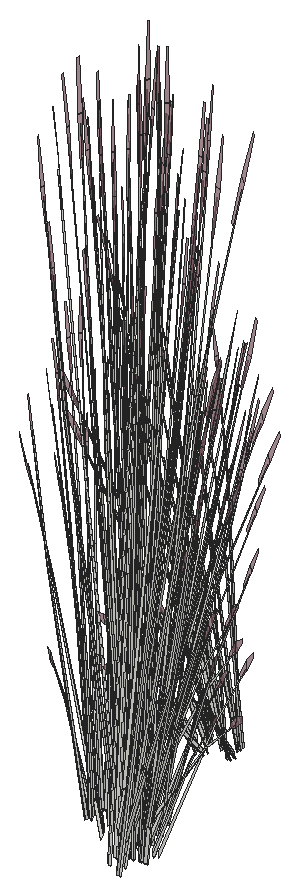
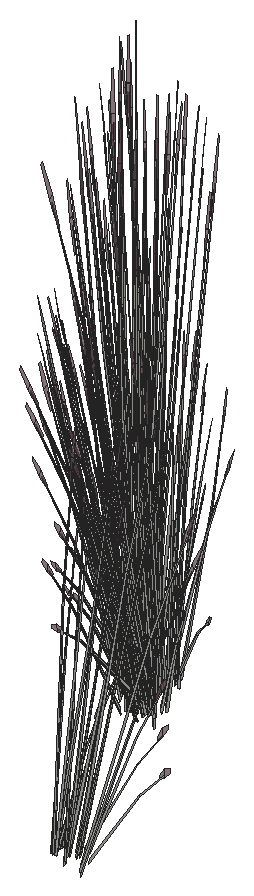
# SketchUp Ruby script. Lengths in inches.
U = 1.inch
M = Sketchup.active_model
def pt(a) = Geom::Point3d.new(a.map { |v| v * U })
def face(e, loops, mat)
  f = e.add_face(loops[0].map { |a| pt(a) })
  loops[1..].each { |l| e.add_face(l.map { |a| pt(a) }).erase! }
  f.material = f.back_material = mat if mat
  f
end
# faces: each face lists its corners as indices into pts; further lists are holes
def faces(e, pts, list, mat = nil) = list.each { |f| face(e, (f[0].is_a?(Array) ? f : [f]).map { |l| l.map { |i| pts[i] } }, mat) }
# xy, xz, yz: faces in a plane at the given z, y or x. An outline is a flat list of corners, or four numbers for a rectangle; further outlines are holes
def ring(l) = l.size == 4 ? [[l[0], l[1]], [l[2], l[1]], [l[2], l[3]], [l[0], l[3]]] : l.each_slice(2).to_a
def flat(e, list, mat, &to3) = list.each { |f| face(e, (f[0].is_a?(Array) ? f : [f]).map { |l| ring(l).map { |u, v| to3.(u, v) } }, mat) }
def xy(e, z, list, mat = nil) = flat(e, list, mat) { |x, y| [x, y, z] }
def xz(e, y, list, mat = nil) = flat(e, list, mat) { |x, z| [x, y, z] }
def yz(e, x, list, mat = nil) = flat(e, list, mat) { |y, z| [x, y, z] }
def lines(e, pts, list) = list.each { |a, b| e.add_line(pt(pts[a]), pt(pts[b])) }
# prism: a flat outline (further loops are holes) pulled along v
def prism(e, loops, v, mat = nil)
  f = face(e, loops, mat); d = Geom::Vector3d.new(v.map { |x| x * U })
  f.pushpull(f.normal.samedirection?(d) ? d.length : -d.length)
end
def box(e, o, s, mat = nil) = prism(e, [[o, [o[0] + s[0], o[1], o[2]], [o[0] + s[0], o[1] + s[1], o[2]], [o[0], o[1] + s[1], o[2]]]], [0, 0, s[2]], mat)
def at(x, y, z, deg = 0) = Geom::Transformation.translation(pt([x, y, z])) * Geom::Transformation.rotation(ORIGIN, Z_AXIS, deg.degrees)
def axes(o, x, y, z) = Geom::Transformation.new([*x, 0, *y, 0, *z, 0, *pt(o).to_a, 1])
def part(name) = M.definitions.add(name)
# library, detail: a bought-in or finely detailed component or shape, given as its bounding box
def library(name, o, s) = part(name).tap { |d| box(d.entities, o, s) }
def detail(e, o, s) = box(e.add_group.entities, o, s)
def put(e, d, t, mat = nil) = e.add_instance(d, t).tap { |i| i.material = mat if mat }
def group(e, t, mat = nil) = e.add_group.tap { |g| g.transformation = t; g.material = mat if mat }.entities
root = M.entities
M.materials.add("LightPink_Translucent").color = [144, 107, 117]
M.materials["LightPink_Translucent"].alpha = 0.75
c1 = part("blade")
p = [[2.15,0.21,22],[0,0.17,0],[0.09,0.45,0],[2.18,0.31,22],[2.29,0.31,22],[0.38,0.45,0],
  [2.48,0.24,33],[2.49,0.24,33],[2.48,0.22,33]]
faces(c1.entities,p,[[0,1,2,3],[4,5,2,3],[6,3,4,7],[8,0,3,6]])
c2 = part("seeds")
p = [[0.3,-0.1,1.38],[-0.01,-0.03,1.59],[-0.01,-0.03,0.03],[0.14,-0.07,-0.07],[0.29,-0.03,3],[0.15,0.01,3.11]]
faces(c2.entities,p,[[0,1,2,3],[1,0,4,5]],"LightPink_Translucent")
c3 = part("blade with seeds")
put(c3.entities,c1,at(0,0,0))
put(c3.entities,c2,axes([2.4,0.25,30.99],[1.5799,-0.05474,1.17369],[-0.12525,1.92788,0.29478],[-0.07173,-0.02425,1.56792]))
put(root,c3,axes([406.07,308.69,4.74],[-0.08839,-0.48081,-0.26641],[0.35106,-0.13653,0.26641],[-0.07077,-0.05545,1.19518]))
put(root,c3,axes([406.53,308.66,5.13],[0.40434,-0.14646,0.15172],[0.09984,0.54504,0.30174],[-0.03606,-0.07941,1.3795]))
put(root,c3,axes([407.36,306.6,5.29],[0.37992,-0.36634,-0.25022],[0.25264,0.51764,-0.43002],[0.09374,0.05257,1.37348]))
put(root,c3,axes([408.87,307.57,6.89],[0.31272,0.15393,-0.30456],[-0.09121,0.44909,0.39319],[0.1259,-0.04118,0.75234]))
put(root,c3,axes([405.98,308.9,4.74],[-0.35217,-0.2759,-0.427],[0.2105,-0.49473,0],[-0.08021,-0.06284,1.35453]))
put(root,c3,axes([408.32,305.63,4.74],[0.35217,0.2759,-0.427],[-0.2105,0.49473,0],[0.08021,0.06284,1.35453]))
put(root,c3,axes([405.19,306.86,6.89],[-0.31272,-0.15393,-0.30456],[0.09121,-0.44909,0.39319],[-0.1259,0.04118,0.75234]))
put(root,c3,axes([407.65,307.2,4.9],[0.42099,0,0],[0,0.57126,0],[0,0,1.5343]))
put(root,c3,axes([406.93,307.92,5.29],[-0.37992,0.36634,-0.25022],[-0.25264,-0.51764,-0.43002],[-0.09374,-0.05257,1.37348]))
put(root,c3,axes([407.77,305.87,5.13],[-0.40434,0.14646,0.15172],[-0.09984,-0.54504,0.30174],[0.03606,0.07941,1.3795]))
put(root,c3,axes([408.02,307.01,6.33],[-0.15608,0.0125,1.47384],[0.10354,-0.54165,0.11917],[0.22242,0.0335,0.63005]))
put(root,c3,axes([408.22,305.84,4.74],[0.08839,0.48081,-0.26641],[-0.35106,0.13653,0.26641],[0.07077,0.05545,1.19518]))
put(root,c3,axes([408.82,307.76,7.07],[0.1382,0.37624,0.0553],[-0.25202,0.18416,0.43534],[0.11109,-0.03633,0.66383]))
put(root,c3,axes([407.51,306.91,5.05],[-0.4756,-0.11626,0.42311],[0.09679,-0.6566,0.16603],[0.0695,0.0634,1.46899]))
put(root,c3,axes([408.8,307.625,7.07],[-0.10631,0.50312,0.41282],[-0.34951,-0.17204,0.34039],[0.13745,-0.03024,0.85423]))
put(root,c3,axes([407.13,308.53,4.9],[-0.12277,-0.47573,0],[0.35059,-0.1666,0],[0,0,1.32759]))
put(root,c3,axes([406.9,308.08,5.25],[-0.07259,0.49245,0.12452],[-0.35466,-0.08548,-0.35559],[-0.06454,-0.05057,1.09]))
put(root,c3,axes([405.52,306.81,7.34],[0.31272,0.15393,0.30456],[-0.09121,0.44909,-0.39319],[-0.1259,0.04118,0.75234]))
put(root,c3,axes([407.59,308.47,4.88],[0.39505,-0.18722,-0.1651],[0.13882,0.53931,0.00007],[0.04361,-0.02069,1.49552]))
put(root,c3,axes([407.73,308.69,5.13],[0.1087,-0.54839,0.15172],[0.39778,0.15519,0.30174],[-0.06871,0.00267,1.3795]))
put(root,c3,axes([407.64,307.45,4.9],[0.26266,0.35642,0],[-0.26266,0.35642,0],[0,0,1.45569]))
put(root,c3,axes([406.15,306.78,5.875],[0.10696,-0.07982,1.52275],[0.03688,0.55733,0.11917],[-0.23167,0.07395,0.54424]))
put(root,c3,axes([408.35,307.29,5.13],[-0.29564,-0.40194,0.15172],[0.29793,-0.38985,0.30174],[-0.03265,0.08208,1.3795]))
put(root,c3,axes([407.8,306.6875,4.77],[0.39143,0.09047,-0.53624],[-0.0826,0.55804,-0.14074],[0.11681,0.06762,1.18365]))
put(root,c3,axes([409.53,307.66,5.38],[-0.23249,0.0911,0.9878],[0.10944,-0.37648,0.72577],[0.12334,0.02576,0.21757]))
put(root,c3,axes([407.05,308.75,4.89],[-0.37935,-0.24773,0],[0.18257,-0.51475,0],[0,0,1.39928]))
put(root,c3,axes([407.36,308.09,5.12],[-0.36743,-0.44413,-0.21665],[0.30918,-0.49872,0.47412],[-0.09894,0.05195,1.44665]))
put(root,c3,axes([406.39,308.94,5.13],[0.35217,0.2759,0.427],[-0.2105,0.49473,0],[-0.08021,-0.06284,1.35453]))
put(root,c3,axes([407.63,307.03,5.34],[0.18257,-0.49721,0.38476],[0.37935,0.23929,-0.18517],[0,0.11462,1.23533]))
put(root,c3,axes([409.42,309.25,7.05],[-0.03403,-0.04831,1.5255],[0.07443,-0.51782,-0.14414],[0.13402,-0.03308,0.26996]))
put(root,c3,axes([405,307.15,7.05],[-0.06145,0.07164,1.50452],[0.00523,0.52344,-0.23794],[-0.14085,0.06807,0.12066]))
put(root,c3,axes([407.56,307.32,4.97],[0,0.63816,-0.04848],[-0.47052,0,0],[0,0.02005,1.54256]))
put(root,c3,axes([405.41,307.08,7.03],[-0.10194,0.50193,-0.43945],[-0.34951,-0.17204,-0.34039],[-0.14072,0.04602,0.84085]))
put(root,c3,axes([405.39,306.65,7.33],[0.18933,0.49965,-0.10458],[-0.33602,0.24554,-0.58045],[-0.1416,0.06592,0.88199]))
put(root,c3,axes([407.6,306.86,4.9],[0.22605,0.46315,-0.38476],[-0.34239,0.32614,0.18517],[0.07315,0.05731,1.23533]))
put(root,c3,axes([409.13,308.82,6.38],[-0.07202,-0.46385,-0.03003],[0.3404,-0.10664,-0.13615],[0.07108,0.02941,0.44908]))
put(root,c3,axes([406.19,309.23,5.04],[-0.23526,0.55293,0],[-0.3936,-0.30836,-0.44382],[-0.08964,-0.07023,1.40792]))
put(root,c3,axes([408.25,308.81,7.33],[0.02015,-0.56117,-0.10458],[0.38148,0.01534,-0.58045],[0.14692,0.03898,0.88199]))
put(root,c3,axes([408.59,307.31,5.13],[0,-0.5518,0.427],[0.42099,0,0],[0,0.12568,1.35453]))
put(root,c3,axes([407.54,307.72,5.34],[0.40861,-0.03406,0.38476],[0.03695,0.56543,-0.18517],[-0.07315,0.05731,1.23533]))
put(root,c3,axes([407.79,307.15,5.25],[0.35059,-0.16092,0.12452],[0.12277,0.45952,-0.35559],[0,0.10113,1.09]))
put(root,c3,axes([408.1875,308.59,7.34],[-0.2141,-0.34548,0.30456],[0.24447,-0.32704,-0.39319],[0.12421,0.04976,0.75234]))
put(root,c3,axes([407.17,308,4.9],[-0.40861,0.03406,-0.38476],[-0.03695,-0.56543,0.18517],[-0.07315,0.05731,1.23533]))
put(root,c3,axes([409.1,308.27,5.23],[-0.09062,-0.13571,1.22981],[0.11791,-0.44895,-0.26449],[0.18335,0.06082,0.52581]))
put(root,c3,axes([407.48,308.76,4.9],[0.37935,0.24773,0],[-0.18257,0.51475,0],[0,0,1.5046]))
put(root,c3,axes([408.58,308.47,7.05],[0.08072,-0.00933,1.50452],[0.22141,-0.42869,-0.23794],[0.14358,0.05659,0.12066]))
put(root,c3,axes([407.63,309.31,4.89],[-0.23233,-0.55486,-0.04422],[0.3936,-0.30836,0.44382],[-0.09699,0.05283,1.40722]))
put(root,c3,axes([407.55,307.97,5.25],[0.278,0.33153,0.12452],[-0.23189,0.37404,-0.35559],[-0.06454,0.05057,1.09]))
put(root,c3,axes([405.35,308.05,7.07],[-0.09332,-0.50785,0.41282],[0.36608,-0.08814,0.34039],[-0.10789,0.11944,0.85423]))
put(root,c3,axes([405.28,307.95,7.07],[-0.25832,-0.23207,0.0553],[0.1504,-0.33047,0.43534],[-0.08282,0.10684,0.66383]))
put(root,c3,axes([405.4,307.34,6.33],[0.13056,-0.11672,1.47384],[0.10992,0.53933,0.11917],[-0.20497,0.12189,0.63005]))
put(root,c3,axes([408.26,308.54,7.28],[0.37615,0.01329,-0.61099],[-0.02526,0.55946,0.07373],[0.15935,0.05904,0.8643]))
put(root,c3,axes([407.84,308.99,5.13],[0.35217,-0.2759,0.427],[0.2105,0.49473,0],[-0.08021,0.06284,1.35453]))
put(root,c3,axes([407.34,308.55,4.97],[0.1636,0.63392,-0.05171],[-0.46745,0.22213,0],[0.00571,0.02214,1.48069]))
put(root,c3,axes([407.52,309.24,4.74],[-0.35106,-0.13653,-0.26641],[0.08839,-0.48081,0.26641],[-0.07077,0.05545,1.19518]))
put(root,c3,axes([404.99,308.26,5.23],[0.13077,0.0453,1.22981],[0.08428,0.46268,-0.26449],[-0.17763,0.08661,0.52581]))
put(root,c3,axes([405.57,307.88,7.34],[0.32754,-0.07886,0.30456],[0.08649,0.45081,-0.39319],[-0.09386,0.12109,0.75234]))
put(root,c3,axes([408.88,307.4,5.04],[0.47052,0,0],[0,0.61671,-0.44382],[0,0.14046,1.40792]))
put(root,c3,axes([404.3125,307.68,7.05],[0.04802,0.0148,1.5255],[0.14856,0.48754,-0.14414],[-0.0983,0.12796,0.26996]))
put(root,c3,axes([408.69,307.72,4.89],[-0.47029,-0.00441,-0.0428],[0,-0.61671,0.42951],[-0.01478,0.14039,1.36183]))
put(root,c3,axes([407.67,307.18,5.29],[0.42377,0.26329,-0.25022],[-0.20405,0.55571,-0.43002],[0.01332,0.13644,1.37348]))
put(root,c3,axes([404.72,309.23,5.38],[0.15682,-0.25009,0.9878],[0.06188,0.39591,0.72577],[-0.11333,0.07089,0.21757]))
put(root,c3,axes([408.49,308.77,6.89],[0.2141,0.34548,-0.30456],[-0.24447,0.32704,0.39319],[0.12421,0.04976,0.75234]))
put(root,c3,axes([408.59,307.81,4.74],[-0.26266,0.34428,-0.26641],[-0.26266,-0.34428,0.26641],[0,0.11089,1.19518]))
put(root,c3,axes([407.46,307.84,5.29],[0.04385,0.62963,-0.25022],[-0.45669,0.03807,-0.43002],[-0.08042,0.08387,1.37348]))
put(root,c3,axes([408.38,308.9,7.07],[-0.01895,0.4196,0.0553],[-0.28611,-0.0115,0.43534],[0.1096,0.04391,0.66383]))
put(root,c3,axes([407.63,307.6,4.9],[-0.18257,0.49721,-0.38476],[-0.37935,-0.23929,0.18517],[0,0.11462,1.23533]))
put(root,c3,axes([405.31,308.15,6.89],[-0.32754,0.07886,-0.30456],[-0.08649,-0.45081,0.39319],[-0.09386,0.12109,0.75234]))
put(root,c3,axes([408.41,308.77,7.07],[-0.27746,0.36359,0.41282],[-0.23929,-0.38612,0.34039],[0.13017,0.06707,0.85423]))
put(root,c3,axes([404.83,309.16,7.86],[0.33205,0.14729,-0.05579],[-0.10214,0.45334,-0.25298],[-0.05431,0.06883,0.83441]))
put(root,c3,axes([407.1875,308.32,4.77],[-0.25345,0.41475,-0.53624],[-0.31485,-0.37608,-0.14074],[-0.10156,0.10346,1.18365]))
put(root,c3,axes([407.53,309.1875,7.34],[-0.05812,-0.44446,0.30456],[0.33222,-0.11736,-0.39319],[0.08923,0.12737,0.75234]))
put(root,c3,axes([407.64,309.02,5],[0.47108,0.17935,0.2645],[-0.11785,0.64108,-0.31383],[-0.07797,0.08023,1.41801]))
put(root,c3,axes([407.6,309.46,4.74],[-0.35217,0.2759,-0.427],[-0.2105,-0.49473,0],[-0.08021,0.06284,1.35453]))
put(root,c3,axes([408.77,307.82,4.74],[0,0.5518,-0.427],[-0.42099,0,0],[0,0.12568,1.35453]))
put(root,c3,axes([407.72,307.88,6.33],[-0.13977,-0.09507,1.47384],[0.28925,-0.39884,0.11917],[0.18028,0.17992,0.63005]))
put(root,c3,axes([407.75,306.63,6.85],[-0.32515,-0.2867,1.18923],[0.34333,-0.44639,0.51312],[0.10491,0.26901,1.1495]))
put(root,c3,axes([405.4,307.84,7.33],[0.34807,0.30426,-0.10458],[-0.20053,0.44063,-0.58045],[-0.09834,0.15317,0.88199]))
put(root,c3,axes([408.24,308.97,5.38],[-0.21187,-0.15866,0.9878],[0.27357,-0.16121,0.72577],[0.07379,0.13656,0.21757]))
put(root,c3,axes([407.49,309.42,7.33],[0.22423,-0.47232,-0.10458],[0.32472,0.27211,-0.58045],[0.11288,0.13344,0.88199]))
put(root,c3,axes([405.875,307.71,6.33],[0.09398,-0.16955,1.47384],[0.23731,0.45764,0.11917],[-0.16276,0.20841,0.63005]))
put(root,c3,axes([405.58,308.2,7.03],[0.09666,0.50384,-0.43945],[-0.36608,0.08814,-0.34039],[-0.10491,0.13533,0.84085]))
put(root,c3,axes([406.02,308.78,7.34],[0.2546,-0.29052,0.30456],[0.24101,0.33173,-0.39319],[-0.03667,0.16855,0.75234]))
put(root,c3,axes([407.92,309.37,5.04],[0.23526,0.55293,0],[-0.3936,0.30836,-0.44382],[-0.08964,0.07023,1.40792]))
put(root,c3,axes([407.2,309.8125,7.05],[0.00111,-0.06681,1.5255],[0.32247,-0.29474,-0.14414],[0.11201,0.1052,0.26996]))
put(root,c3,axes([408.3,309.56,4.28],[0.02741,-0.07966,1.51654],[0.34514,-0.23462,-0.23168],[0.10464,0.12143,0.25832]))
put(root,c3,axes([407.72,307.18,5.44],[-0.01028,-0.51954,1.21494],[0.46521,0.13467,0.51441],[-0.11003,0.28429,1.14681]))
put(root,c3,axes([407.84,307.75,4.8],[0.13798,0.50522,-0.59522],[-0.39745,0.18195,-0.15622],[0.01525,0.17108,1.31385]))
put(root,c3,axes([405.79,309.05,7.07],[-0.30922,-0.02571,0.0553],[0.00848,-0.38824,0.43534],[-0.03236,0.14872,0.66383]))
put(root,c3,axes([405.13,309.49,4.28],[0.05047,0.05513,1.51654],[0.08558,0.51079,-0.23168],[-0.11187,0.10892,0.25832]))
put(root,c3,axes([405.88,309.08,7.07],[-0.26795,-0.37649,0.41282],[0.28456,-0.3247,0.34039],[-0.04943,0.17664,0.85423]))
put(root,c3,axes([407.76,309.18,7.03],[0.37131,-0.13117,-0.43945],[0.06495,0.49674,-0.34039],[0.09973,0.14235,0.84085]))
put(root,c3,axes([406.73,309.26,7.34],[0.11344,-0.42434,0.30456],[0.33096,0.12377,-0.39319],[0.03035,0.17085,0.75234]))
put(root,c3,axes([408.27,309.6875,5.29],[-0.2413,-0.01731,0.90352],[0.15935,-0.36755,0.49885],[0.09532,0.13058,0.70873]))
put(root,c3,axes([407.58,309.59,7.07],[-0.17102,0.35053,0.0553],[-0.24354,-0.20408,0.43534],[0.07874,0.11238,0.66383]))
put(root,c3,axes([407.18,310.77,7.86],[0.26003,-0.31656,-0.05579],[0.23826,0.3467,-0.25298],[0.01677,0.09824,0.83441]))
put(root,c3,axes([407.65,309.49,7.07],[-0.37426,0.12663,0.41282],[-0.06495,-0.49674,0.34039],[0.08802,0.1464,0.85423]))
put(root,c3,axes([405.8,308.125,6.33],[0.07006,-0.18966,1.47384],[0.29392,0.3925,0.11917],[-0.13259,0.24463,0.63005]))
put(root,c3,axes([407.48,308.8,5.23],[0.00664,-0.18292,1.22981],[0.31732,-0.20432,-0.26449],[0.09796,0.21893,0.52581]))
put(root,c3,axes([406.63,309.64,7.07],[-0.27727,0.18753,0.0553],[-0.13571,-0.34197,0.43534],[0.02678,0.15075,0.66383]))
put(root,c3,axes([405.88,309.19,6.89],[-0.2546,0.29052,-0.30456],[-0.24101,-0.33173,0.39319],[-0.03667,0.16855,0.75234]))
put(root,c3,axes([405.01,309.11,7.05],[-0.00935,0.1092,1.50452],[0.26544,0.37987,-0.23794],[-0.06949,0.17964,0.12066]))
put(root,c3,axes([405.85,308.86,7.64],[0.41355,0.02734,-0.11608],[-0.0113,0.51765,-0.6443],[-0.02873,0.19937,0.97901]))
put(root,c3,axes([406.62,309.4375,7.33],[0.36822,-0.25691,-0.10458],[0.18095,0.45596,-0.58045],[0.04858,0.19215,0.88199]))
put(root,c3,axes([406.73,309.61,7.35],[-0.37078,-0.14426,0.45823],[0.12679,-0.47426,0.37783],[0.02228,0.18651,0.9482]))
put(root,c3,axes([406.05,310.32,5.38],[-0.00974,-0.3281,0.9878],[0.24334,0.23402,0.72577],[-0.04786,0.15639,0.21757]))
put(root,c3,axes([406.6875,309.54,4.28],[0.0609,-0.03003,1.51654],[0.36632,0.16527,-0.23168],[0.01071,0.18627,0.25832]))
put(root,c3,axes([406.14,309.06,7.3],[0.26937,0.37076,-0.48779],[-0.28456,0.3247,-0.37783],[-0.04099,0.18838,0.93334]))
put(root,c3,axes([405.84,309.61,5.43],[0.34184,-0.09771,0.05596],[0.07859,0.39367,-0.74222],[-0.02167,0.19928,0.6653]))
put(root,c3,axes([406.9375,309.42,7.03],[0.3699,0.13833,-0.43945],[-0.12679,0.47426,-0.34039],[0.03392,0.19095,0.84085]))
put(root,c3,axes([407.15,308.4375,6.33],[-0.08601,-0.17716,1.47384],[0.39746,-0.14915,0.11917],[0.08983,0.27813,0.63005]))
put(root,c3,axes([406.77,309.71,6.89],[-0.11344,0.42434,-0.30456],[-0.33096,-0.12377,0.39319],[0.03035,0.17085,0.75234]))
put(root,c3,axes([406.05,308.89,7.59],[-0.00979,0.51041,-0.6782],[-0.4123,-0.03428,0.08184],[-0.04351,0.21623,0.95938]))
put(root,c3,axes([404.98,310.23,7.05],[0.04269,-0.03331,1.5255],[0.35284,0.2216,-0.14414],[-0.00829,0.1845,0.26996]))
put(root,c3,axes([406.44,308.52,6.33],[-0.00921,-0.21179,1.47384],[0.39917,0.1405,0.11917],[-0.02469,0.30182,0.63005]))
put(root,c3,axes([406.8,309.33,7.28],[0.17959,0.44867,-0.61099],[-0.36969,0.25004,0.07373],[0.042,0.21679,0.8643]))
put(root,c3,axes([405.76,310.03,5.23],[0.11874,-0.08705,1.22981],[0.29317,0.26247,-0.26449],[-0.08726,0.22711,0.52581]))
put(root,c3,axes([406.53,310.46,7.05],[0.0477,0.08886,1.50452],[0.38493,0.03491,-0.23794],[0.03871,0.19596,0.12066]))
put(root,c3,axes([405.92,309.61,5.89],[0.00827,-0.28486,1.32737],[0.37184,0.15046,0.18343],[-0.03222,0.30359,0.62678]))
put(root,c3,axes([399.65,325.0625,1.33],[0.08601,0.17716,1.47384],[-0.39746,0.14915,0.11917],[-0.08983,-0.27813,0.63005]))
put(root,c3,axes([400.31,323.89,2.05],[-0.05755,-0.07737,1.50452],[-0.38409,0.04905,-0.23794],[-0.0613,-0.18505,0.12066]))
put(root,c3,axes([402.03,324.84,2.05],[-0.00363,-0.10982,1.50452],[-0.30678,-0.3174,-0.23794],[0.04743,-0.1924,0.12066]))
put(root,c3,axes([400.99,325.375,1.33],[-0.07006,0.18966,1.47384],[-0.29392,-0.3925,0.11917],[0.13259,-0.24463,0.63005]))
put(root,c3,axes([401.95,324.44,2.05],[-0.03821,0.04215,1.5255],[-0.37441,-0.1422,-0.14414],[-0.01355,-0.18393,0.26996]))
put(root,c3,axes([399.91,323.64,2.05],[-0.00702,0.06614,1.5255],[-0.34622,0.24004,-0.14414],[-0.10188,-0.1227,0.26996]))
put(root,c3,axes([399.84,324.81,2.38],[0.41917,-0.14183,0.46236],[0.07275,0.55635,0.38124],[-0.09858,-0.16397,0.95674]))
put(root,c3,axes([400.79,324.91,2.07],[0.37078,0.14426,0.41282],[-0.12679,0.47426,0.34039],[-0.02228,-0.18651,0.85423]))
put(root,c3,axes([400.89,325.08,2.33],[-0.36822,0.25691,-0.10458],[-0.18095,-0.45596,-0.58045],[-0.04858,-0.19215,0.88199]))
put(root,c3,axes([401.66,325.66,2.33],[-0.41355,-0.02734,-0.10458],[0.0113,-0.51765,-0.58045],[0.02873,-0.19937,0.88199]))
put(root,c3,axes([400.88,324.88,2.07],[0.27727,-0.18753,0.0553],[0.13571,0.34197,0.43534],[-0.02678,-0.15075,0.66383]))
put(root,c3,axes([399.93,324.93,2.07],[0.17102,-0.35053,0.0553],[0.24354,0.20408,0.43534],[-0.07874,-0.11238,0.66383]))
put(root,c3,axes([399.08,325.62,1.33],[0.13977,0.09507,1.47384],[-0.28925,0.39884,0.11917],[-0.18028,-0.17992,0.63005]))
put(root,c3,axes([400.78,325.26,2.34],[-0.11344,0.42434,0.30456],[-0.33096,-0.12377,-0.39319],[-0.03035,-0.17085,0.75234]))
put(root,c3,axes([401.63,325.44,2.07],[0.26795,0.37649,0.41282],[-0.28456,0.3247,0.34039],[0.04943,-0.17664,0.85423]))
put(root,c3,axes([400.01,324.89,2.67],[-0.25113,0.52899,-0.11713],[-0.36369,-0.30476,-0.65011],[-0.12642,-0.14945,0.98783]))
put(root,c3,axes([401.73,325.48,2.07],[0.30922,0.02571,0.0553],[-0.00848,0.38824,0.43534],[0.03236,-0.14872,0.66383]))
put(root,c3,axes([401.49,325.74,2.34],[-0.2546,0.29052,0.30456],[-0.24101,-0.33173,-0.39319],[0.03667,-0.16855,0.75234]))
put(root,c3,axes([399.05,324.74,2.05],[-0.08096,-0.00389,1.50452],[-0.25776,0.38949,-0.23794],[-0.13753,-0.07958,0.12066]))
